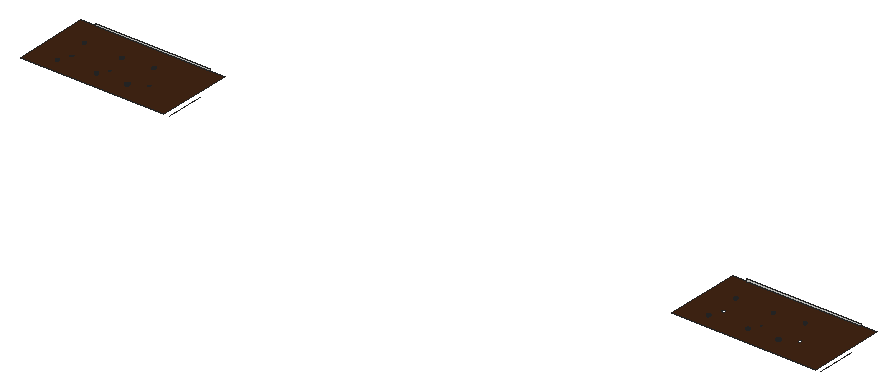
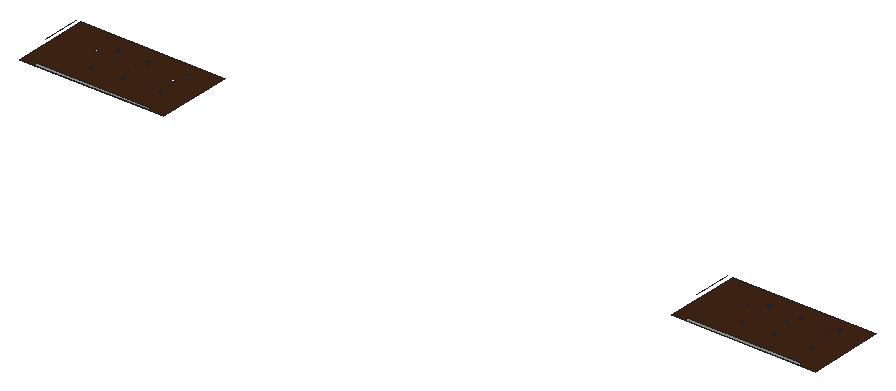
# SketchUp Ruby script. Lengths in inches.
U = 1.inch
M = Sketchup.active_model
def pt(a) = Geom::Point3d.new(a.map { |v| v * U })
def face(e, loops, mat)
  f = e.add_face(loops[0].map { |a| pt(a) })
  loops[1..].each { |l| e.add_face(l.map { |a| pt(a) }).erase! }
  f.material = f.back_material = mat if mat
  f
end
# faces: each face lists its corners as indices into pts; further lists are holes
def faces(e, pts, list, mat = nil) = list.each { |f| face(e, (f[0].is_a?(Array) ? f : [f]).map { |l| l.map { |i| pts[i] } }, mat) }
# xy, xz, yz: faces in a plane at the given z, y or x. An outline is a flat list of corners, or four numbers for a rectangle; further outlines are holes
def ring(l) = l.size == 4 ? [[l[0], l[1]], [l[2], l[1]], [l[2], l[3]], [l[0], l[3]]] : l.each_slice(2).to_a
def flat(e, list, mat, &to3) = list.each { |f| face(e, (f[0].is_a?(Array) ? f : [f]).map { |l| ring(l).map { |u, v| to3.(u, v) } }, mat) }
def xy(e, z, list, mat = nil) = flat(e, list, mat) { |x, y| [x, y, z] }
def xz(e, y, list, mat = nil) = flat(e, list, mat) { |x, z| [x, y, z] }
def yz(e, x, list, mat = nil) = flat(e, list, mat) { |y, z| [x, y, z] }
def lines(e, pts, list) = list.each { |a, b| e.add_line(pt(pts[a]), pt(pts[b])) }
# prism: a flat outline (further loops are holes) pulled along v
def prism(e, loops, v, mat = nil)
  f = face(e, loops, mat); d = Geom::Vector3d.new(v.map { |x| x * U })
  f.pushpull(f.normal.samedirection?(d) ? d.length : -d.length)
end
def box(e, o, s, mat = nil) = prism(e, [[o, [o[0] + s[0], o[1], o[2]], [o[0] + s[0], o[1] + s[1], o[2]], [o[0], o[1] + s[1], o[2]]]], [0, 0, s[2]], mat)
def at(x, y, z, deg = 0) = Geom::Transformation.translation(pt([x, y, z])) * Geom::Transformation.rotation(ORIGIN, Z_AXIS, deg.degrees)
def axes(o, x, y, z) = Geom::Transformation.new([*x, 0, *y, 0, *z, 0, *pt(o).to_a, 1])
def part(name) = M.definitions.add(name)
# library, detail: a bought-in or finely detailed component or shape, given as its bounding box
def library(name, o, s) = part(name).tap { |d| box(d.entities, o, s) }
def detail(e, o, s) = box(e.add_group.entities, o, s)
def put(e, d, t, mat = nil) = e.add_instance(d, t).tap { |i| i.material = mat if mat }
def group(e, t, mat = nil) = e.add_group.tap { |g| g.transformation = t; g.material = mat if mat }.entities
root = M.entities
M.materials.add("[Field Square Tile]").color = [211, 167, 108]
M.materials.add("[Wood Veneer 01]").color = [66, 38, 20]
xy(root,251.5,[[[232.96,458.5,427.1,561.05],[273.1,492.27,273.89,492.375,274.63,492.68,275.26,493.17,275.75,493.8,276.06,494.54,276.16,495.33,276.06,496.125,275.75,496.86,275.26,497.5,274.63,497.98,273.89,498.29,273.1,498.39,272.31,498.29,271.57,497.98,270.93,497.5,270.45,496.86,270.14,496.125,270.04,495.33,270.14,494.54,270.45,493.8,270.93,493.17,271.57,492.68,272.31,492.375],[377.04,492.58,377.75,492.68,378.42,492.95,378.99,493.39,379.42,493.96,379.7,494.62,379.79,495.33,379.7,496.04,379.42,496.71,378.99,497.28,378.42,497.71,377.75,497.99,377.04,498.08,376.33,497.99,375.67,497.71,375.1,497.28,374.66,496.71,374.39,496.04,374.29,495.33,374.39,494.62,374.66,493.96,375.1,493.39,375.67,492.95,376.33,492.68],[324.47,492.77,325.13,492.86,325.75,493.11,326.28,493.52,326.69,494.05,326.95,494.67,327.03,495.33,326.95,495.99,326.69,496.61,326.28,497.14,325.75,497.55,325.13,497.81,324.47,497.89,323.81,497.81,323.19,497.55,322.66,497.14,322.25,496.61,322,495.99,321.91,495.33,322,494.67,322.25,494.05,322.66,493.52,323.19,493.11,323.81,492.86],[357.2,481.02,357.83,481.11,358.42,481.35,358.92,481.74,359.31,482.24,359.55,482.83,359.63,483.46,359.55,484.09,359.31,484.68,358.92,485.18,358.42,485.57,357.83,485.8125,357.2,485.9,356.57,485.8125,355.98,485.57,355.47,485.18,355.09,484.68,354.84,484.09,354.76,483.46,354.84,482.83,355.09,482.24,355.47,481.74,355.98,481.35,356.57,481.11],[266.8,522.58,267.28,522.64,267.74,522.83,268.125,523.13,268.42,523.52,268.61,523.97,268.67,524.45,268.61,524.94,268.42,525.39,268.125,525.78,267.74,526.08,267.28,526.27,266.8,526.33,266.3125,526.27,265.86,526.08,265.47,525.78,265.17,525.39,264.99,524.94,264.92,524.45,264.99,523.97,265.17,523.52,265.47,523.13,265.86,522.83,266.3125,522.64],[317.24,522.58,317.72,522.64,318.17,522.83,318.5625,523.13,318.86,523.52,319.05,523.97,319.11,524.45,319.05,524.94,318.86,525.39,318.5625,525.78,318.17,526.08,317.72,526.27,317.24,526.33,316.75,526.27,316.3,526.08,315.91,525.78,315.61,525.39,315.42,524.94,315.36,524.45,315.42,523.97,315.61,523.52,315.91,523.13,316.3,522.83,316.75,522.64],[317.24,479.77,317.72,479.83,318.17,480.02,318.5625,480.32,318.86,480.7,319.05,481.16,319.11,481.64,319.05,482.13,318.86,482.58,318.5625,482.97,318.17,483.27,317.72,483.45,317.24,483.52,316.75,483.45,316.3,483.27,315.91,482.97,315.61,482.58,315.42,482.13,315.36,481.64,315.42,481.16,315.61,480.7,315.91,480.32,316.3,480.02,316.75,479.83],[266.8,476.64,267.28,476.71,267.74,476.89,268.125,477.19,268.42,477.58,268.61,478.03,268.67,478.52,268.61,479,268.42,479.45,268.125,479.84,267.74,480.14,267.28,480.33,266.8,480.39,266.3125,480.33,265.86,480.14,265.47,479.84,265.17,479.45,264.99,479,264.92,478.52,264.99,478.03,265.17,477.58,265.47,477.19,265.86,476.89,266.3125,476.71],[357.2,526.75,357.63,526.8125,358.04,526.98,358.39,527.25,358.66,527.6,358.83,528,358.88,528.44,358.83,528.88,358.66,529.28,358.39,529.63,358.04,529.9,357.63,530.07,357.2,530.13,356.76,530.07,356.35,529.9,356,529.63,355.74,529.28,355.57,528.88,355.51,528.44,355.57,528,355.74,527.6,356,527.25,356.35,526.98,356.76,526.8125]],[[1111.71,458.5,1305.85,561.05],[1151.85,492.27,1152.64,492.375,1153.38,492.68,1154.01,493.17,1154.5,493.8,1154.81,494.54,1154.91,495.33,1154.81,496.125,1154.5,496.86,1154.01,497.5,1153.38,497.98,1152.64,498.29,1151.85,498.39,1151.06,498.29,1150.32,497.98,1149.68,497.5,1149.2,496.86,1148.89,496.125,1148.79,495.33,1148.89,494.54,1149.2,493.8,1149.68,493.17,1150.32,492.68,1151.06,492.375],[1255.79,492.58,1256.5,492.68,1257.17,492.95,1257.74,493.39,1258.17,493.96,1258.45,494.62,1258.54,495.33,1258.45,496.04,1258.17,496.71,1257.74,497.28,1257.17,497.71,1256.5,497.99,1255.79,498.08,1255.08,497.99,1254.42,497.71,1253.85,497.28,1253.41,496.71,1253.14,496.04,1253.04,495.33,1253.14,494.62,1253.41,493.96,1253.85,493.39,1254.42,492.95,1255.08,492.68],[1203.22,492.77,1203.88,492.86,1204.5,493.11,1205.03,493.52,1205.44,494.05,1205.7,494.67,1205.78,495.33,1205.7,495.99,1205.44,496.61,1205.03,497.14,1204.5,497.55,1203.88,497.81,1203.22,497.89,1202.56,497.81,1201.94,497.55,1201.41,497.14,1201,496.61,1200.75,495.99,1200.66,495.33,1200.75,494.67,1201,494.05,1201.41,493.52,1201.94,493.11,1202.56,492.86],[1235.95,481.02,1236.58,481.11,1237.17,481.35,1237.67,481.74,1238.06,482.24,1238.3,482.83,1238.38,483.46,1238.3,484.09,1238.06,484.68,1237.67,485.18,1237.17,485.57,1236.58,485.8125,1235.95,485.9,1235.32,485.8125,1234.73,485.57,1234.22,485.18,1233.84,484.68,1233.59,484.09,1233.51,483.46,1233.59,482.83,1233.84,482.24,1234.22,481.74,1234.73,481.35,1235.32,481.11],[1145.55,522.58,1146.03,522.64,1146.49,522.83,1146.875,523.13,1147.17,523.52,1147.36,523.97,1147.42,524.45,1147.36,524.94,1147.17,525.39,1146.875,525.78,1146.49,526.08,1146.03,526.27,1145.55,526.33,1145.0625,526.27,1144.61,526.08,1144.22,525.78,1143.92,525.39,1143.74,524.94,1143.67,524.45,1143.74,523.97,1143.92,523.52,1144.22,523.13,1144.61,522.83,1145.0625,522.64],[1195.99,522.58,1196.47,522.64,1196.92,522.83,1197.3125,523.13,1197.61,523.52,1197.8,523.97,1197.86,524.45,1197.8,524.94,1197.61,525.39,1197.3125,525.78,1196.92,526.08,1196.47,526.27,1195.99,526.33,1195.5,526.27,1195.05,526.08,1194.66,525.78,1194.36,525.39,1194.17,524.94,1194.11,524.45,1194.17,523.97,1194.36,523.52,1194.66,523.13,1195.05,522.83,1195.5,522.64],[1195.99,479.77,1196.47,479.83,1196.92,480.02,1197.3125,480.32,1197.61,480.7,1197.8,481.16,1197.86,481.64,1197.8,482.13,1197.61,482.58,1197.3125,482.97,1196.92,483.27,1196.47,483.45,1195.99,483.52,1195.5,483.45,1195.05,483.27,1194.66,482.97,1194.36,482.58,1194.17,482.13,1194.11,481.64,1194.17,481.16,1194.36,480.7,1194.66,480.32,1195.05,480.02,1195.5,479.83],[1145.55,476.64,1146.03,476.71,1146.49,476.89,1146.875,477.19,1147.17,477.58,1147.36,478.03,1147.42,478.52,1147.36,479,1147.17,479.45,1146.875,479.84,1146.49,480.14,1146.03,480.33,1145.55,480.39,1145.0625,480.33,1144.61,480.14,1144.22,479.84,1143.92,479.45,1143.74,479,1143.67,478.52,1143.74,478.03,1143.92,477.58,1144.22,477.19,1144.61,476.89,1145.0625,476.71],[1235.95,526.75,1236.38,526.8125,1236.79,526.98,1237.14,527.25,1237.41,527.6,1237.58,528,1237.63,528.44,1237.58,528.88,1237.41,529.28,1237.14,529.63,1236.79,529.9,1236.38,530.07,1235.95,530.13,1235.51,530.07,1235.1,529.9,1234.75,529.63,1234.49,529.28,1234.32,528.88,1234.26,528.44,1234.32,528,1234.49,527.6,1234.75,527.25,1235.1,526.98,1235.51,526.8125]]],"[Wood Veneer 01]")
xz(root,561.05,[[252.78,251.5,252.84,254.5],[252.84,251.5,406.85,254.5],[1131.53,251.5,1131.59,254.5],[1131.59,251.5,1285.6,254.5]])
p = [[266.8,476.64,251.5],[266.3125,476.71,251.5],[266.3125,476.71,252.5],[266.8,476.64,252.5],[267.28,476.71,251.5],[267.28,476.71,252.5],
  [1145.55,476.64,251.5],[1145.0625,476.71,251.5],[1145.0625,476.71,252.5],[1145.55,476.64,252.5],[1146.03,476.71,251.5],[1146.03,476.71,252.5],
  [265.86,476.89,251.5],[265.86,476.89,252.5],[267.74,476.89,251.5],[267.74,476.89,252.5],[1144.61,476.89,251.5],[1144.61,476.89,252.5],
  [1146.49,476.89,251.5],[1146.49,476.89,252.5],[265.47,477.19,251.5],[265.47,477.19,252.5],[268.125,477.19,251.5],[268.125,477.19,252.5],
  [1144.22,477.19,251.5],[1144.22,477.19,252.5],[1146.875,477.19,251.5],[1146.875,477.19,252.5],[265.17,477.58,251.5],[265.17,477.58,252.5],
  [268.42,477.58,251.5],[268.42,477.58,252.5],[1143.92,477.58,251.5],[1143.92,477.58,252.5],[1147.17,477.58,251.5],[1147.17,477.58,252.5],
  [264.99,478.03,251.5],[264.99,478.03,252.5],[268.61,478.03,251.5],[268.61,478.03,252.5],[1143.74,478.03,251.5],[1143.74,478.03,252.5],
  [1147.36,478.03,251.5],[1147.36,478.03,252.5],[264.92,478.52,251.5],[264.92,478.52,252.5],[268.67,478.52,251.5],[268.67,478.52,252.5],
  [1143.67,478.52,251.5],[1143.67,478.52,252.5],[1147.42,478.52,251.5],[1147.42,478.52,252.5],[264.99,479,251.5],[264.99,479,252.5],
  [268.61,479,251.5],[268.61,479,252.5],[1143.74,479,251.5],[1143.74,479,252.5],[1147.36,479,251.5],[1147.36,479,252.5],
  [265.17,479.45,251.5],[265.17,479.45,252.5],[268.42,479.45,251.5],[268.42,479.45,252.5],[1143.92,479.45,251.5],[1143.92,479.45,252.5],
  [1147.17,479.45,251.5],[1147.17,479.45,252.5],[265.47,479.84,251.5],[265.47,479.84,252.5],[268.125,479.84,251.5],[268.125,479.84,252.5],
  [1144.22,479.84,251.5],[1144.22,479.84,252.5],[1146.875,479.84,251.5],[1146.875,479.84,252.5],[265.86,480.14,251.5],[265.86,480.14,252.5],
  [267.74,480.14,251.5],[267.74,480.14,252.5],[316.75,479.83,251.5],[316.3,480.02,251.5],[316.3,480.02,252.5],[316.75,479.83,252.5],
  [317.24,479.77,251.5],[317.24,479.77,252.5],[317.72,479.83,251.5],[317.72,479.83,252.5],[318.17,480.02,251.5],[318.17,480.02,252.5],
  [1144.61,480.14,251.5],[1144.61,480.14,252.5],[1146.49,480.14,251.5],[1146.49,480.14,252.5],[1195.5,479.83,251.5],[1195.05,480.02,251.5],
  [1195.05,480.02,252.5],[1195.5,479.83,252.5],[1195.99,479.77,251.5],[1195.99,479.77,252.5],[1196.47,479.83,251.5],[1196.47,479.83,252.5],
  [1196.92,480.02,251.5],[1196.92,480.02,252.5],[315.91,480.32,251.5],[315.91,480.32,252.5],[318.5625,480.32,251.5],[318.5625,480.32,252.5],
  [1194.66,480.32,251.5],[1194.66,480.32,252.5],[1197.3125,480.32,251.5],[1197.3125,480.32,252.5],[266.3125,480.33,251.5],[266.3125,480.33,252.5],
  [267.28,480.33,251.5],[267.28,480.33,252.5],[1145.0625,480.33,251.5],[1145.0625,480.33,252.5],[1146.03,480.33,251.5],[1146.03,480.33,252.5],
  [266.8,480.39,251.5],[266.8,480.39,252.5],[315.61,480.7,251.5],[315.61,480.7,252.5],[318.86,480.7,251.5],[318.86,480.7,252.5],
  [1145.55,480.39,251.5],[1145.55,480.39,252.5],[1194.36,480.7,251.5],[1194.36,480.7,252.5],[1197.61,480.7,251.5],[1197.61,480.7,252.5],
  [315.42,481.16,251.5],[315.42,481.16,252.5],[319.05,481.16,251.5],[319.05,481.16,252.5],[1194.17,481.16,251.5],[1194.17,481.16,252.5],
  [1197.8,481.16,251.5],[1197.8,481.16,252.5],[357.2,481.02,251.5],[356.57,481.11,251.5],[356.57,481.11,252.5625],[357.2,481.02,252.5625],
  [357.83,481.11,251.5],[357.83,481.11,252.5625],[1235.95,481.02,251.5],[1235.32,481.11,251.5],[1235.32,481.11,252.5625],[1235.95,481.02,252.5625],
  [1236.58,481.11,251.5],[1236.58,481.11,252.5625],[355.98,481.35,251.5],[355.98,481.35,252.5625],[358.42,481.35,251.5],[358.42,481.35,252.5625],
  [1234.73,481.35,251.5],[1234.73,481.35,252.5625],[1237.17,481.35,251.5],[1237.17,481.35,252.5625],[315.36,481.64,251.5],[315.36,481.64,252.5],
  [319.11,481.64,251.5],[319.11,481.64,252.5],[1194.11,481.64,251.5],[1194.11,481.64,252.5],[1197.86,481.64,251.5],[1197.86,481.64,252.5],
  [355.47,481.74,251.5],[355.47,481.74,252.5625],[358.92,481.74,251.5],[358.92,481.74,252.5625],[1234.22,481.74,251.5],[1234.22,481.74,252.5625],
  [1237.67,481.74,251.5],[1237.67,481.74,252.5625],[315.42,482.13,251.5],[315.42,482.13,252.5],[319.05,482.13,251.5],[319.05,482.13,252.5],
  [1194.17,482.13,251.5],[1194.17,482.13,252.5],[1197.8,482.13,251.5],[1197.8,482.13,252.5],[355.09,482.24,251.5],[355.09,482.24,252.5625],
  [359.31,482.24,251.5],[359.31,482.24,252.5625],[1233.84,482.24,251.5],[1233.84,482.24,252.5625],[1238.06,482.24,251.5],[1238.06,482.24,252.5625],
  [315.61,482.58,251.5],[315.61,482.58,252.5],[318.86,482.58,251.5],[318.86,482.58,252.5],[1194.36,482.58,251.5],[1194.36,482.58,252.5],
  [1197.61,482.58,251.5],[1197.61,482.58,252.5],[354.84,482.83,251.5],[354.84,482.83,252.5625],[359.55,482.83,251.5],[359.55,482.83,252.5625],
  [1233.59,482.83,251.5],[1233.59,482.83,252.5625],[1238.3,482.83,251.5],[1238.3,482.83,252.5625],[315.91,482.97,251.5],[315.91,482.97,252.5],
  [318.5625,482.97,251.5],[318.5625,482.97,252.5],[1194.66,482.97,251.5],[1194.66,482.97,252.5],[1197.3125,482.97,251.5],[1197.3125,482.97,252.5],
  [354.76,483.46,251.5],[354.76,483.46,252.5625],[359.63,483.46,251.5],[359.63,483.46,252.5625],[1233.51,483.46,251.5],[1233.51,483.46,252.5625],
  [1238.38,483.46,251.5],[1238.38,483.46,252.5625],[316.3,483.27,251.5],[316.3,483.27,252.5],[318.17,483.27,251.5],[318.17,483.27,252.5],
  [1195.05,483.27,251.5],[1195.05,483.27,252.5],[1196.92,483.27,251.5],[1196.92,483.27,252.5],[316.75,483.45,251.5],[316.75,483.45,252.5],
  [317.72,483.45,251.5],[317.72,483.45,252.5],[1195.5,483.45,251.5],[1195.5,483.45,252.5],[1196.47,483.45,251.5],[1196.47,483.45,252.5],
  [317.24,483.52,251.5],[317.24,483.52,252.5],[354.84,484.09,251.5],[354.84,484.09,252.5625],[359.55,484.09,251.5],[359.55,484.09,252.5625],
  [1195.99,483.52,251.5],[1195.99,483.52,252.5],[1233.59,484.09,251.5],[1233.59,484.09,252.5625],[1238.3,484.09,251.5],[1238.3,484.09,252.5625],
  [355.09,484.68,251.5],[355.09,484.68,252.5625],[359.31,484.68,251.5],[359.31,484.68,252.5625],[1233.84,484.68,251.5],[1233.84,484.68,252.5625],
  [1238.06,484.68,251.5],[1238.06,484.68,252.5625],[355.47,485.18,251.5],[355.47,485.18,252.5625],[358.92,485.18,251.5],[358.92,485.18,252.5625],
  [1234.22,485.18,251.5],[1234.22,485.18,252.5625],[1237.67,485.18,251.5],[1237.67,485.18,252.5625],[355.98,485.57,251.5],[355.98,485.57,252.5625],
  [358.42,485.57,251.5],[358.42,485.57,252.5625],[1234.73,485.57,251.5],[1234.73,485.57,252.5625],[1237.17,485.57,251.5],[1237.17,485.57,252.5625],
  [356.57,485.8125,251.5],[356.57,485.8125,252.5625],[357.83,485.8125,251.5],[357.83,485.8125,252.5625],[1235.32,485.8125,251.5],[1235.32,485.8125,252.5625],
  [1236.58,485.8125,251.5],[1236.58,485.8125,252.5625],[357.2,485.9,251.5],[357.2,485.9,252.5625],[1235.95,485.9,251.5],[1235.95,485.9,252.5625],
  [266.3125,522.64,251.5],[265.86,522.83,251.5],[265.86,522.83,252.5],[266.3125,522.64,252.5],[266.8,522.58,251.5],[266.8,522.58,252.5],
  [267.28,522.64,251.5],[267.28,522.64,252.5],[267.74,522.83,251.5],[267.74,522.83,252.5],[316.75,522.64,251.5],[316.3,522.83,251.5],
  [316.3,522.83,252.5],[316.75,522.64,252.5],[317.24,522.58,251.5],[317.24,522.58,252.5],[317.72,522.64,251.5],[317.72,522.64,252.5],
  [318.17,522.83,251.5],[318.17,522.83,252.5],[1145.0625,522.64,251.5],[1144.61,522.83,251.5],[1144.61,522.83,252.5],[1145.0625,522.64,252.5],
  [1145.55,522.58,251.5],[1145.55,522.58,252.5],[1146.03,522.64,251.5],[1146.03,522.64,252.5],[1146.49,522.83,251.5],[1146.49,522.83,252.5],
  [1195.5,522.64,251.5],[1195.05,522.83,251.5],[1195.05,522.83,252.5],[1195.5,522.64,252.5],[1195.99,522.58,251.5],[1195.99,522.58,252.5],
  [1196.47,522.64,251.5],[1196.47,522.64,252.5],[1196.92,522.83,251.5],[1196.92,522.83,252.5],[265.47,523.13,251.5],[265.47,523.13,252.5],
  [268.125,523.13,251.5],[268.125,523.13,252.5],[315.91,523.13,251.5],[315.91,523.13,252.5],[318.5625,523.13,251.5],[318.5625,523.13,252.5],
  [1144.22,523.13,251.5],[1144.22,523.13,252.5],[1146.875,523.13,251.5],[1146.875,523.13,252.5],[1194.66,523.13,251.5],[1194.66,523.13,252.5],
  [1197.3125,523.13,251.5],[1197.3125,523.13,252.5],[265.17,523.52,251.5],[265.17,523.52,252.5],[268.42,523.52,251.5],[268.42,523.52,252.5],
  [315.61,523.52,251.5],[315.61,523.52,252.5],[318.86,523.52,251.5],[318.86,523.52,252.5],[1143.92,523.52,251.5],[1143.92,523.52,252.5],
  [1147.17,523.52,251.5],[1147.17,523.52,252.5],[1194.36,523.52,251.5],[1194.36,523.52,252.5],[1197.61,523.52,251.5],[1197.61,523.52,252.5],
  [264.99,523.97,251.5],[264.99,523.97,252.5],[268.61,523.97,251.5],[268.61,523.97,252.5],[315.42,523.97,251.5],[315.42,523.97,252.5],
  [319.05,523.97,251.5],[319.05,523.97,252.5],[1143.74,523.97,251.5],[1143.74,523.97,252.5],[1147.36,523.97,251.5],[1147.36,523.97,252.5],
  [1194.17,523.97,251.5],[1194.17,523.97,252.5],[1197.8,523.97,251.5],[1197.8,523.97,252.5],[264.92,524.45,251.5],[264.92,524.45,252.5],
  [268.67,524.45,251.5],[268.67,524.45,252.5],[315.36,524.45,251.5],[315.36,524.45,252.5],[319.11,524.45,251.5],[319.11,524.45,252.5],
  [1143.67,524.45,251.5],[1143.67,524.45,252.5],[1147.42,524.45,251.5],[1147.42,524.45,252.5],[1194.11,524.45,251.5],[1194.11,524.45,252.5],
  [1197.86,524.45,251.5],[1197.86,524.45,252.5],[264.99,524.94,251.5],[264.99,524.94,252.5],[268.61,524.94,251.5],[268.61,524.94,252.5],
  [315.42,524.94,251.5],[315.42,524.94,252.5],[319.05,524.94,251.5],[319.05,524.94,252.5],[1143.74,524.94,251.5],[1143.74,524.94,252.5],
  [1147.36,524.94,251.5],[1147.36,524.94,252.5],[1194.17,524.94,251.5],[1194.17,524.94,252.5],[1197.8,524.94,251.5],[1197.8,524.94,252.5],
  [265.17,525.39,251.5],[265.17,525.39,252.5],[268.42,525.39,251.5],[268.42,525.39,252.5],[315.61,525.39,251.5],[315.61,525.39,252.5],
  [318.86,525.39,251.5],[318.86,525.39,252.5],[1143.92,525.39,251.5],[1143.92,525.39,252.5],[1147.17,525.39,251.5],[1147.17,525.39,252.5],
  [1194.36,525.39,251.5],[1194.36,525.39,252.5],[1197.61,525.39,251.5],[1197.61,525.39,252.5],[265.47,525.78,251.5],[265.47,525.78,252.5],
  [268.125,525.78,251.5],[268.125,525.78,252.5],[315.91,525.78,251.5],[315.91,525.78,252.5],[318.5625,525.78,251.5],[318.5625,525.78,252.5],
  [1144.22,525.78,251.5],[1144.22,525.78,252.5],[1146.875,525.78,251.5],[1146.875,525.78,252.5],[1194.66,525.78,251.5],[1194.66,525.78,252.5],
  [1197.3125,525.78,251.5],[1197.3125,525.78,252.5],[265.86,526.08,251.5],[265.86,526.08,252.5],[267.74,526.08,251.5],[267.74,526.08,252.5],
  [316.3,526.08,251.5],[316.3,526.08,252.5],[318.17,526.08,251.5],[318.17,526.08,252.5],[1144.61,526.08,251.5],[1144.61,526.08,252.5],
  [1146.49,526.08,251.5],[1146.49,526.08,252.5],[1195.05,526.08,251.5],[1195.05,526.08,252.5],[1196.92,526.08,251.5],[1196.92,526.08,252.5],
  [266.3125,526.27,251.5],[266.3125,526.27,252.5],[267.28,526.27,251.5],[267.28,526.27,252.5],[316.75,526.27,251.5],[316.75,526.27,252.5],
  [317.72,526.27,251.5],[317.72,526.27,252.5],[1145.0625,526.27,251.5],[1145.0625,526.27,252.5],[1146.03,526.27,251.5],[1146.03,526.27,252.5],
  [1195.5,526.27,251.5],[1195.5,526.27,252.5],[1196.47,526.27,251.5],[1196.47,526.27,252.5],[266.8,526.33,251.5],[266.8,526.33,252.5],
  [317.24,526.33,251.5],[317.24,526.33,252.5],[1145.55,526.33,251.5],[1145.55,526.33,252.5],[1195.99,526.33,251.5],[1195.99,526.33,252.5],
  [356.76,526.8125,251.5],[356.35,526.98,251.5],[356.35,526.98,252.4375],[356.76,526.8125,252.4375],[357.2,526.75,251.5],[357.2,526.75,252.4375],
  [357.63,526.8125,251.5],[357.63,526.8125,252.4375],[358.04,526.98,251.5],[358.04,526.98,252.4375],[1235.51,526.8125,251.5],[1235.1,526.98,251.5],
  [1235.1,526.98,252.4375],[1235.51,526.8125,252.4375],[1235.95,526.75,251.5],[1235.95,526.75,252.4375],[1236.38,526.8125,251.5],[1236.38,526.8125,252.4375],
  [1236.79,526.98,251.5],[1236.79,526.98,252.4375],[356,527.25,251.5],[356,527.25,252.4375],[358.39,527.25,251.5],[358.39,527.25,252.4375],
  [1234.75,527.25,251.5],[1234.75,527.25,252.4375],[1237.14,527.25,251.5],[1237.14,527.25,252.4375],[355.74,527.6,251.5],[355.74,527.6,252.4375],
  [358.66,527.6,251.5],[358.66,527.6,252.4375],[1234.49,527.6,251.5],[1234.49,527.6,252.4375],[1237.41,527.6,251.5],[1237.41,527.6,252.4375],
  [355.57,528,251.5],[355.57,528,252.4375],[358.83,528,251.5],[358.83,528,252.4375],[1234.32,528,251.5],[1234.32,528,252.4375],
  [1237.58,528,251.5],[1237.58,528,252.4375],[355.51,528.44,251.5],[355.51,528.44,252.4375],[358.88,528.44,251.5],[358.88,528.44,252.4375],
  [1234.26,528.44,251.5],[1234.26,528.44,252.4375],[1237.63,528.44,251.5],[1237.63,528.44,252.4375],[355.57,528.88,251.5],[355.57,528.88,252.4375],
  [358.83,528.88,251.5],[358.83,528.88,252.4375],[1234.32,528.88,251.5],[1234.32,528.88,252.4375],[1237.58,528.88,251.5],[1237.58,528.88,252.4375],
  [355.74,529.28,251.5],[355.74,529.28,252.4375],[358.66,529.28,251.5],[358.66,529.28,252.4375],[1234.49,529.28,251.5],[1234.49,529.28,252.4375],
  [1237.41,529.28,251.5],[1237.41,529.28,252.4375],[356,529.63,251.5],[356,529.63,252.4375],[358.39,529.63,251.5],[358.39,529.63,252.4375],
  [1234.75,529.63,251.5],[1234.75,529.63,252.4375],[1237.14,529.63,251.5],[1237.14,529.63,252.4375],[356.35,529.9,251.5],[356.35,529.9,252.4375],
  [358.04,529.9,251.5],[358.04,529.9,252.4375],[1235.1,529.9,251.5],[1235.1,529.9,252.4375],[1236.79,529.9,251.5],[1236.79,529.9,252.4375],
  [356.76,530.07,251.5],[356.76,530.07,252.4375],[357.63,530.07,251.5],[357.63,530.07,252.4375],[1235.51,530.07,251.5],[1235.51,530.07,252.4375],
  [1236.38,530.07,251.5],[1236.38,530.07,252.4375],[357.2,530.13,251.5],[357.2,530.13,252.4375],[1235.95,530.13,251.5],[1235.95,530.13,252.4375],
  [433.97,511.08,251.5],[433.97,458.5,251.5],[1312.72,511.08,251.5],[1312.72,458.5,251.5]]
faces(root,p,[[0,1,2,3],[4,0,3,5],[6,7,8,9],[10,6,9,11],[1,12,13,2],[14,4,5,15],[7,16,17,8],[18,10,11,19],
  [12,20,21,13],[22,14,15,23],[16,24,25,17],[26,18,19,27],[20,28,29,21],[30,22,23,31],[24,32,33,25],[34,26,27,35],
  [28,36,37,29],[38,30,31,39],[32,40,41,33],[42,34,35,43],[36,44,45,37],[46,38,39,47],[40,48,49,41],[50,42,43,51],
  [44,52,53,45],[54,46,47,55],[48,56,57,49],[58,50,51,59],[52,60,61,53],[62,54,55,63],[56,64,65,57],[66,58,59,67],
  [60,68,69,61],[70,62,63,71],[64,72,73,65],[74,66,67,75],[68,76,77,69],[78,70,71,79],[80,81,82,83],[84,80,83,85],
  [86,84,85,87],[88,86,87,89],[72,90,91,73],[92,74,75,93],[94,95,96,97],[98,94,97,99],[100,98,99,101],[102,100,101,103],
  [81,104,105,82],[106,88,89,107],[95,108,109,96],[110,102,103,111],[76,112,113,77],[114,78,79,115],[90,116,117,91],[118,92,93,119],
  [112,120,121,113],[120,114,115,121],[104,122,123,105],[124,106,107,125],[116,126,127,117],[126,118,119,127],[108,128,129,109],[130,110,111,131],
  [122,132,133,123],[134,124,125,135],[128,136,137,129],[138,130,131,139],[140,141,142,143],[144,140,143,145],[146,147,148,149],[150,146,149,151],
  [141,152,153,142],[154,144,145,155],[147,156,157,148],[158,150,151,159],[132,160,161,133],[162,134,135,163],[136,164,165,137],[166,138,139,167],
  [152,168,169,153],[170,154,155,171],[156,172,173,157],[174,158,159,175],[160,176,177,161],[178,162,163,179],[164,180,181,165],[182,166,167,183],
  [168,184,185,169],[186,170,171,187],[172,188,189,173],[190,174,175,191],[176,192,193,177],[194,178,179,195],[180,196,197,181],[198,182,183,199],
  [184,200,201,185],[202,186,187,203],[188,204,205,189],[206,190,191,207],[192,208,209,193],[210,194,195,211],[196,212,213,197],[214,198,199,215],
  [200,216,217,201],[218,202,203,219],[204,220,221,205],[222,206,207,223],[208,224,225,209],[226,210,211,227],[212,228,229,213],[230,214,215,231],
  [224,232,233,225],[234,226,227,235],[228,236,237,229],[238,230,231,239],[232,240,241,233],[240,234,235,241],[216,242,243,217],[244,218,219,245],
  [236,246,247,237],[246,238,239,247],[220,248,249,221],[250,222,223,251],[242,252,253,243],[254,244,245,255],[248,256,257,249],[258,250,251,259],
  [252,260,261,253],[262,254,255,263],[256,264,265,257],[266,258,259,267],[260,268,269,261],[270,262,263,271],[264,272,273,265],[274,266,267,275],
  [268,276,277,269],[278,270,271,279],[272,280,281,273],[282,274,275,283],[276,284,285,277],[284,278,279,285],[280,286,287,281],[286,282,283,287],
  [288,289,290,291],[292,288,291,293],[294,292,293,295],[296,294,295,297],[298,299,300,301],[302,298,301,303],[304,302,303,305],[306,304,305,307],
  [308,309,310,311],[312,308,311,313],[314,312,313,315],[316,314,315,317],[318,319,320,321],[322,318,321,323],[324,322,323,325],[326,324,325,327],
  [289,328,329,290],[330,296,297,331],[299,332,333,300],[334,306,307,335],[309,336,337,310],[338,316,317,339],[319,340,341,320],[342,326,327,343],
  [328,344,345,329],[346,330,331,347],[332,348,349,333],[350,334,335,351],[336,352,353,337],[354,338,339,355],[340,356,357,341],[358,342,343,359],
  [344,360,361,345],[362,346,347,363],[348,364,365,349],[366,350,351,367],[352,368,369,353],[370,354,355,371],[356,372,373,357],[374,358,359,375],
  [360,376,377,361],[378,362,363,379],[364,380,381,365],[382,366,367,383],[368,384,385,369],[386,370,371,387],[372,388,389,373],[390,374,375,391],
  [376,392,393,377],[394,378,379,395],[380,396,397,381],[398,382,383,399],[384,400,401,385],[402,386,387,403],[388,404,405,389],[406,390,391,407],
  [392,408,409,393],[410,394,395,411],[396,412,413,397],[414,398,399,415],[400,416,417,401],[418,402,403,419],[404,420,421,405],[422,406,407,423],
  [408,424,425,409],[426,410,411,427],[412,428,429,413],[430,414,415,431],[416,432,433,417],[434,418,419,435],[420,436,437,421],[438,422,423,439],
  [424,440,441,425],[442,426,427,443],[428,444,445,429],[446,430,431,447],[432,448,449,433],[450,434,435,451],[436,452,453,437],[454,438,439,455],
  [440,456,457,441],[458,442,443,459],[444,460,461,445],[462,446,447,463],[448,464,465,449],[466,450,451,467],[452,468,469,453],[470,454,455,471],
  [456,472,473,457],[472,458,459,473],[460,474,475,461],[474,462,463,475],[464,476,477,465],[476,466,467,477],[468,478,479,469],[478,470,471,479],
  [480,481,482,483],[484,480,483,485],[486,484,485,487],[488,486,487,489],[490,491,492,493],[494,490,493,495],[496,494,495,497],[498,496,497,499],
  [481,500,501,482],[502,488,489,503],[491,504,505,492],[506,498,499,507],[500,508,509,501],[510,502,503,511],[504,512,513,505],[514,506,507,515],
  [508,516,517,509],[518,510,511,519],[512,520,521,513],[522,514,515,523],[516,524,525,517],[526,518,519,527],[520,528,529,521],[530,522,523,531],
  [524,532,533,525],[534,526,527,535],[528,536,537,529],[538,530,531,539],[532,540,541,533],[542,534,535,543],[536,544,545,537],[546,538,539,547],
  [540,548,549,541],[550,542,543,551],[544,552,553,545],[554,546,547,555],[548,556,557,549],[558,550,551,559],[552,560,561,553],[562,554,555,563],
  [556,564,565,557],[566,558,559,567],[560,568,569,561],[570,562,563,571],[564,572,573,565],[572,566,567,573],[568,574,575,569],[574,570,571,575]],"[Field Square Tile]")
lines(root,p,[[576,577],[578,579]])
